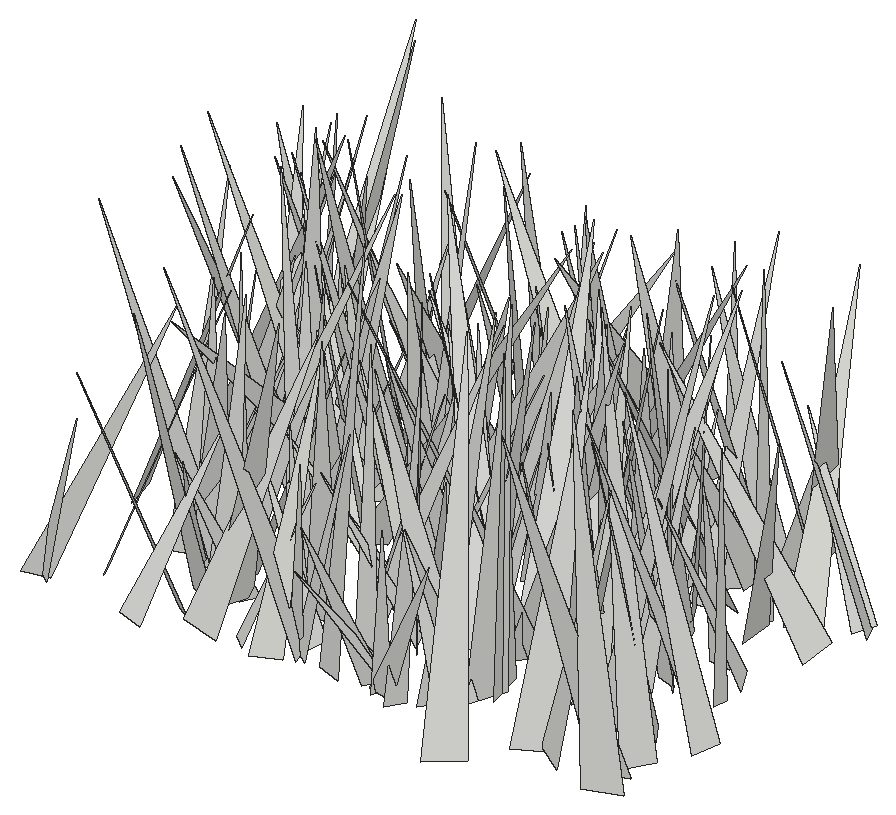
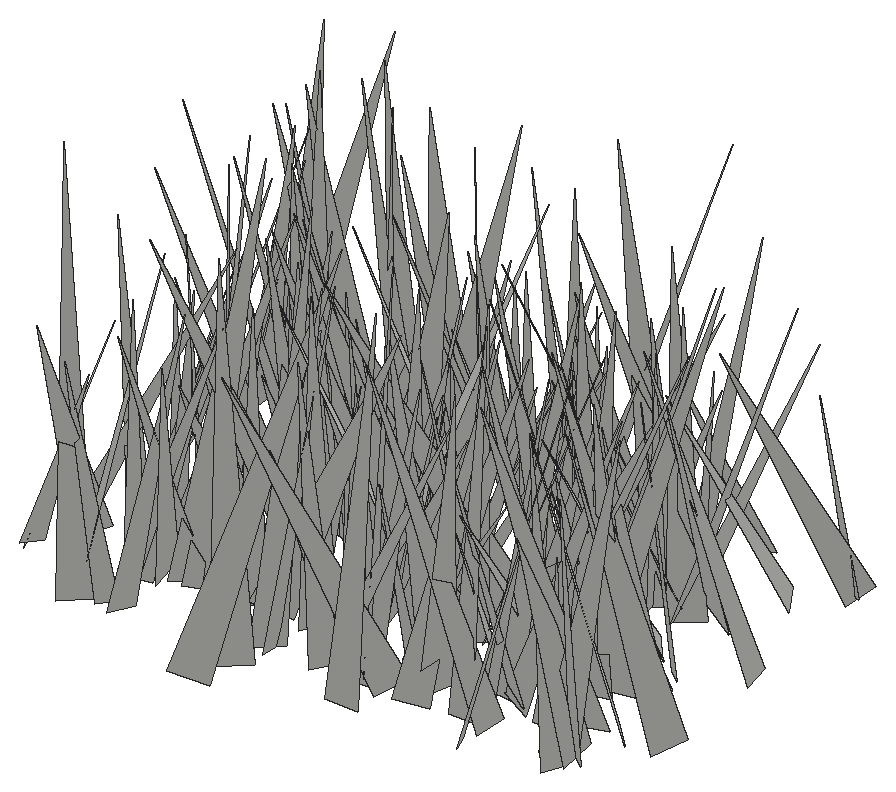
# SketchUp Ruby script. Lengths in inches.
U = 1.inch
M = Sketchup.active_model
def pt(a) = Geom::Point3d.new(a.map { |v| v * U })
def face(e, loops, mat)
  f = e.add_face(loops[0].map { |a| pt(a) })
  loops[1..].each { |l| e.add_face(l.map { |a| pt(a) }).erase! }
  f.material = f.back_material = mat if mat
  f
end
# faces: each face lists its corners as indices into pts; further lists are holes
def faces(e, pts, list, mat = nil) = list.each { |f| face(e, (f[0].is_a?(Array) ? f : [f]).map { |l| l.map { |i| pts[i] } }, mat) }
# xy, xz, yz: faces in a plane at the given z, y or x. An outline is a flat list of corners, or four numbers for a rectangle; further outlines are holes
def ring(l) = l.size == 4 ? [[l[0], l[1]], [l[2], l[1]], [l[2], l[3]], [l[0], l[3]]] : l.each_slice(2).to_a
def flat(e, list, mat, &to3) = list.each { |f| face(e, (f[0].is_a?(Array) ? f : [f]).map { |l| ring(l).map { |u, v| to3.(u, v) } }, mat) }
def xy(e, z, list, mat = nil) = flat(e, list, mat) { |x, y| [x, y, z] }
def xz(e, y, list, mat = nil) = flat(e, list, mat) { |x, z| [x, y, z] }
def yz(e, x, list, mat = nil) = flat(e, list, mat) { |y, z| [x, y, z] }
def lines(e, pts, list) = list.each { |a, b| e.add_line(pt(pts[a]), pt(pts[b])) }
# prism: a flat outline (further loops are holes) pulled along v
def prism(e, loops, v, mat = nil)
  f = face(e, loops, mat); d = Geom::Vector3d.new(v.map { |x| x * U })
  f.pushpull(f.normal.samedirection?(d) ? d.length : -d.length)
end
def box(e, o, s, mat = nil) = prism(e, [[o, [o[0] + s[0], o[1], o[2]], [o[0] + s[0], o[1] + s[1], o[2]], [o[0], o[1] + s[1], o[2]]]], [0, 0, s[2]], mat)
def at(x, y, z, deg = 0) = Geom::Transformation.translation(pt([x, y, z])) * Geom::Transformation.rotation(ORIGIN, Z_AXIS, deg.degrees)
def axes(o, x, y, z) = Geom::Transformation.new([*x, 0, *y, 0, *z, 0, *pt(o).to_a, 1])
def part(name) = M.definitions.add(name)
# library, detail: a bought-in or finely detailed component or shape, given as its bounding box
def library(name, o, s) = part(name).tap { |d| box(d.entities, o, s) }
def detail(e, o, s) = box(e.add_group.entities, o, s)
def put(e, d, t, mat = nil) = e.add_instance(d, t).tap { |i| i.material = mat if mat }
def group(e, t, mat = nil) = e.add_group.tap { |g| g.transformation = t; g.material = mat if mat }.entities
root = M.entities
c1 = part("fur_instance\#9")
p = [[0.8125,0,1.79],[0.67,-0.02,1.48],[0,-0.11,0],[0,0.11,0]]
faces(c1.entities,p,[[0,1,2,3]])
put(root,c1,axes([494.21,43.57,-21.86],[-3.24466,-1.65637,0.06319],[-1.44148,2.88818,1.68993],[0.81834,-1.47993,3.2273]))
put(root,c1,axes([493.82,43.125,-21.86],[1.92833,-3.54748,0.58332],[-3.33012,-2.01195,-1.22706],[-1.35468,-0.10385,3.84674]))
put(root,c1,axes([504.59,43.15,-21.86],[0.14854,-7.36709,1.66817],[-7.40985,-0.46607,-1.39849],[-1.46661,1.60862,7.23466]))
put(root,c1,axes([479.7,41.96,-21.86],[2.1321,2.91958,1.28602],[3.18698,-1.87905,-1.01782],[0.14466,-1.63367,3.46899]))
put(root,c1,axes([494.51,42.625,-21.86],[1.15805,-3.96128,0.43832],[-3.70743,-0.90324,1.63219],[1.46246,0.84697,3.79062]))
put(root,c1,axes([505.06,42.02,-21.86],[1.15068,-6.84996,3.27998],[-7.48842,-1.57649,-0.66528],[-1.26644,3.09791,6.914]))
put(root,c1,axes([490.3,43.63,-21.86],[-7.76303,-2.55675,1.09489],[-2.43873,7.81802,0.96517],[1.33728,-0.58482,8.11604]))
put(root,c1,axes([485.34,42.9,-21.86],[-3.10953,-4.00727,0.37973],[-3.98696,3.00024,-0.98706],[-0.55366,0.90108,4.97525]))
put(root,c1,axes([494.37,42.82,-21.86],[3.31226,-1.52366,0.97308],[-1.49474,-3.45052,-0.31491],[-1.01694,0.10903,3.63228]))
put(root,c1,axes([499.3,40.25,-21.86],[5.53383,-2.65462,5.00816],[-4.23304,-6.59023,1.18414],[-3.76962,3.5034,6.0223]))
put(root,c1,axes([484.17,41.32,-21.86],[0.26684,4.21608,0.5662],[4.07293,-0.08948,-1.25314],[1.22767,-0.6195,4.03438]))
put(root,c1,axes([497.21,43.58,-21.86],[4.68158,-4.31782,3.21331],[-4.18207,-5.59908,-1.43065],[-3.3881,0.94493,6.20597]))
put(root,c1,axes([496.99,44.51,-21.86],[4.08531,-1.79648,1.28746],[-1.24322,-4.1049,-1.78292],[-1.82737,-1.22355,4.09124]))
put(root,c1,axes([485.21,44.25,-21.86],[-2.27159,-6.08211,1.19958],[-6.16809,2.34544,0.21162],[0.62109,1.04786,6.48903]))
put(root,c1,axes([502.05,42.74,-21.86],[3.01267,4.99828,1.819],[5.31773,-2.78497,-1.15474],[0.11548,-2.15148,5.72063]))
put(root,c1,axes([486.27,44.47,-21.86],[7.12513,-3.29011,0.44393],[-3.26274,-7.13377,-0.50321],[-0.6135,-0.27186,7.83192]))
put(root,c1,axes([490.04,43.42,-21.86],[-1.12295,-3.74744,1.45837],[-3.89173,1.39395,0.58526],[1.01223,1.20198,3.86805]))
put(root,c1,axes([486.59,42.27,-21.86],[0.24671,6.36494,1.6516],[6.30189,0.24313,-1.87833],[1.87786,-1.65213,6.08648]))
put(root,c1,axes([488.23,42.47,-21.86],[2.19151,2.85606,0.09461],[2.85445,-2.18225,-0.24214],[0.13471,-0.22234,3.59182]))
put(root,c1,axes([490.47,43.09,-21.86],[2.5994,3.80823,1.24151],[3.99906,-2.55122,-0.54734],[-0.2268,-1.33772,4.57819]))
put(root,c1,axes([479.54,41.77,-21.86],[5.30796,-1.91017,1.71118],[-2.50762,-4.68997,2.54311],[-0.53734,3.01775,5.03546]))
put(root,c1,axes([483.86,45.68,-21.86],[4.12034,-0.14152,0.59374],[0.17297,-3.61498,-2.06197],[-0.58535,-2.06437,3.57009]))
put(root,c1,axes([486.6,45.11,-21.86],[1.61464,-3.26071,0.69447],[-2.99454,-1.75765,-1.29032],[-1.46534,-0.00102,3.40211]))
put(root,c1,axes([489.68,42.16,-21.86],[-4.32625,3.6169,1.13686],[3.35652,4.45591,-1.40339],[1.76301,0.39209,5.46158]))
put(root,c1,axes([490.55,44.03,-21.86],[-3.79909,0.62191,0.11225],[0.62576,3.79759,0.13861],[0.08831,-0.15497,3.84716]))
put(root,c1,axes([495.39,42.34,-21.86],[-6.05732,0.47074,1.68041],[-0.07648,5.99257,-1.95441],[1.74342,1.89841,5.75265]))
put(root,c1,axes([501.28,42.81,-21.86],[-4.71435,5.59524,2.23508],[5.56124,5.13291,-1.11952],[2.31839,-0.93486,7.23039]))
put(root,c1,axes([489.55,45.53,-21.86],[0.93072,-6.54849,1.55591],[-6.7031,-0.75944,0.81335],[0.60996,1.64631,6.5641]))
put(root,c1,axes([492.14,42.65,-21.86],[3.45024,7.01244,2.07893],[6.95776,-3.8555,1.45774],[-2.25516,-1.1667,7.67811]))
put(root,c1,axes([489.56,44.42,-21.86],[0.08392,3.77547,1.67654],[4.10941,-0.2474,0.35143],[-0.42151,-1.66031,3.76001]))
put(root,c1,axes([497.6,44.75,-21.86],[7.52534,-2.11015,2.94691],[-2.32099,-8.02168,0.183],[-2.78389,0.98374,7.81345]))
put(root,c1,axes([496.41,43.25,-21.86],[-6.74927,1.80081,2.69667],[1.18797,7.16726,-1.81295],[3.01723,1.2063,6.74602]))
put(root,c1,axes([497.76,45.6,-21.86],[-6.42267,-1.42598,3.31634],[-1.29179,7.22813,0.60623],[3.37087,0.05298,6.55107]))
put(root,c1,axes([483.23,47.04,-21.86],[3.73638,-5.69312,0.32255],[-5.69521,-3.70663,0.54933],[0.28337,0.57053,6.78752]))
put(root,c1,axes([493.14,46.59,-21.86],[-3.84083,-1.16764,0.10273],[-1.10793,3.73134,0.98769],[0.38264,-0.91633,3.89099]))
put(root,c1,axes([496.77,45.57,-21.86],[7.78387,0.2727,2.09642],[0.3333,-8.05673,-0.18953],[-2.08764,-0.26953,7.78634]))
put(root,c1,axes([492.2,44.7,-21.86],[1.00537,5.49165,1.69021],[5.63183,-1.28199,0.81538],[-1.13911,-1.49133,5.52306]))
put(root,c1,axes([493.0625,46.44,-21.86],[5.50119,4.10651,2.99111],[4.73487,-5.74232,-0.82461],[-1.84151,-2.49711,6.81516]))
put(root,c1,axes([481.34,43.51,-21.86],[4.7893,3.01055,0.30481],[2.77693,-4.59952,1.79634],[-1.20208,1.36921,5.36414]))
put(root,c1,axes([485.07,45.49,-21.86],[4.88657,-1.90502,2.44295],[-2.30886,-5.28158,0.49977],[-2.06549,1.39696,5.22091]))
put(root,c1,axes([503.95,46.5,-21.86],[-4.7875,-3.33897,1.34753],[-3.4677,4.87923,-0.23006],[0.96934,0.96392,5.83232]))
put(root,c1,axes([483.83,46.17,-21.86],[0.33576,5.45677,2.6197],[6.05197,-0.25349,-0.24764],[0.11336,-2.62894,5.46148]))
put(root,c1,axes([483.78,46.71,-21.86],[-7.05109,-1.52018,0.70264],[-1.52291,7.08527,0.04653],[0.69669,0.10238,7.21295]))
put(root,c1,axes([491.65,47.875,-21.86],[-4.59032,-0.23962,0.17171],[-0.16134,4.28449,1.66587],[0.24672,-1.65642,4.28408]))
put(root,c1,axes([505.12,47.69,-21.86],[-6.09562,-2.74651,0.83103],[-2.67616,6.14538,0.68045],[1.03541,-0.28555,6.65108]))
put(root,c1,axes([504.86,44.28,-21.86],[-8.1921,1.36867,0.61461],[1.20152,8.02801,-1.8625],[0.89853,1.74336,8.09413]))
put(root,c1,axes([497.72,47.76,-21.86],[-0.21744,-4.53269,0.61909],[-4.46943,0.07824,-0.99696],[-0.9761,0.65149,4.42703]))
put(root,c1,axes([484.6875,46.88,-21.86],[0.05129,-4.93553,2.34933],[-4.99892,0.90807,2.01684],[2.21125,2.16734,4.50493]))
put(root,c1,axes([491.35,45.6875,-21.86],[3.76049,3.04894,0.61025],[2.98388,-3.80785,0.6375],[-0.87456,0.11813,4.79905]))
put(root,c1,axes([491.22,46.125,-21.86],[3.55811,5.92159,0.8478],[5.93377,-3.36884,-1.37307],[0.75783,-1.4247,6.77052]))
put(root,c1,axes([497.4,50.3,-21.86],[1.43301,-8.2393,0.15598],[-8.02359,-1.35888,1.93375],[1.87948,0.48092,8.13635]))
put(root,c1,axes([506.01,46.69,-21.86],[-6.67851,0.63047,0.27765],[0.60623,6.66388,-0.54986],[0.32721,0.52189,6.68563]))
put(root,c1,axes([485.01,46.55,-21.86],[-5.66532,-0.50223,1.85308],[-0.88322,5.80808,-1.12609],[1.70472,1.34012,5.57494]))
put(root,c1,axes([485.65,46.37,-21.86],[4.63443,1.21877,0.59299],[1.09033,-4.6073,0.94811],[-0.80513,0.77609,4.69728]))
put(root,c1,axes([496.93,47.83,-21.86],[7.07738,-3.29601,0.99897],[-3.4049,-7.03943,0.89669],[-0.51794,1.23844,7.75557]))
put(root,c1,axes([492.52,47.16,-21.86],[5.45999,3.37552,0.2587],[3.37248,-5.38033,-0.97518],[0.29572,-0.96459,6.34466]))
put(root,c1,axes([498.69,49.59,-21.86],[1.50872,-5.62418,0.24688],[-5.60162,-1.47433,0.64555],[0.56049,0.40439,5.78713]))
put(root,c1,axes([491.5,49.68,-21.86],[-0.15941,-4.26775,0.08772],[-3.87813,0.18147,1.78158],[1.78369,0.01316,3.88138]))
put(root,c1,axes([492.75,49.84,-21.86],[1.73584,-5.70606,0.92261],[-5.63591,-1.88469,-1.0526],[-1.28332,0.55882,5.87063]))
put(root,c1,axes([502.09,45.85,-21.86],[3.85814,7.37241,1.12129],[7.37277,-3.96052,0.67189],[-1.11889,-0.67587,8.29374]))
put(root,c1,axes([493.59,51.07,-21.86],[-5.30348,-5.59312,0.1785],[-5.55783,5.29332,0.73008],[0.65218,-0.37354,7.67313]))
put(root,c1,axes([487.97,46.46,-21.86],[-7.72963,0.57294,0.92033],[0.30078,7.49944,-2.14251],[1.04153,2.08628,7.44883]))
put(root,c1,axes([491.89,48.14,-21.86],[-4.67921,0.76999,0.1435],[0.76372,4.67821,-0.1991],[0.17382,0.17327,4.73796]))
put(root,c1,axes([500.125,46.79,-21.86],[6.4621,3.38539,1.99868],[3.00841,-6.73382,1.67909],[-2.53082,0.63956,7.09931]))
put(root,c1,axes([484.01,46.44,-21.86],[4.66085,6.54813,0.11631],[6.5407,-4.64683,-0.4912],[0.3329,-0.37945,8.02249]))
put(root,c1,axes([485.61,53.69,-21.86],[5.32765,-5.22538,0.29084],[-4.03169,-4.36253,-4.52625],[-3.33686,-3.07194,5.93309]))
put(root,c1,axes([482.48,46.23,-21.86],[2.16067,6.65454,0.44246],[6.23565,-2.18071,2.34697],[-2.36543,0.32979,6.59114]))
put(root,c1,axes([495.39,47.69,-21.86],[-5.00695,6.61488,0.9269],[6.67749,4.92855,0.89773],[-0.16413,-1.27989,8.24744]))
put(root,c1,axes([478.77,48.67,-21.86],[6.39935,1.66924,0.57136],[1.67346,-6.42366,0.02366],[-0.55885,-0.12123,6.61343]))
put(root,c1,axes([486.08,50.76,-21.86],[1.95757,-4.55386,0.31612],[-4.56359,-1.94437,0.25034],[0.10577,0.38911,4.95045]))
put(root,c1,axes([494.55,48.66,-21.86],[-0.54447,5.56352,1.73211],[5.79599,0.33809,0.73596],[-0.59958,-1.78391,5.54144]))
put(root,c1,axes([501.86,49.64,-21.86],[-2.15143,-4.58063,1.63472],[-4.86135,2.07952,-0.57094],[0.14745,1.72526,5.02841]))
put(root,c1,axes([496.65,49.89,-21.86],[-1.9321,-3.03286,0.9193],[-3.13143,1.99261,-0.00754],[0.48737,0.77951,3.596]))
put(root,c1,axes([493.47,50.32,-21.86],[3.99613,2.0991,0.80323],[2.24013,-3.58697,-1.77087],[0.18236,-1.93595,4.15203]))
put(root,c1,axes([501.96,49.77,-21.86],[4.37424,4.04681,2.79179],[4.54542,-4.75288,-0.23239],[-1.87347,-2.08284,5.95454]))
put(root,c1,axes([484.71,50.74,-21.86],[-7.47727,-2.4998,1.10622],[-2.44373,7.5564,0.55783],[1.22512,-0.18436,7.86431]))
put(root,c1,axes([495.05,48.03,-21.86],[-1.19348,5.65379,0.3473],[5.3271,0.99964,2.033],[-1.92561,-0.73875,5.40894]))
put(root,c1,axes([503.95,51.41,-21.86],[-4.09527,-2.1175,0.66115],[-1.87882,4.04889,1.32991],[1.17939,-0.90267,4.41434]))
put(root,c1,axes([485.18,50.01,-21.86],[5.23095,-0.44242,1.6949],[-0.413,-5.49862,-0.16069],[-1.70231,-0.02548,5.24716]))
put(root,c1,axes([482.97,52.85,-21.86],[-1.44964,-7.72306,0.36058],[-7.72764,1.4358,-0.315],[-0.24346,0.41228,7.85162]))
put(root,c1,axes([481.11,50.42,-21.86],[3.62429,3.41254,1.71474],[3.78655,-3.51895,-1.00013],[-0.49783,-1.92166,4.87654]))
put(root,c1,axes([497.43,52.25,-21.86],[5.27759,-3.33069,0.22963],[-3.2336,-5.20637,-1.19863],[-0.83073,-0.89406,6.12452]))
put(root,c1,axes([488.09,50.05,-21.86],[-3.65286,-4.07637,1.60167],[-4.37583,3.48496,-1.11027],[0.18514,1.94004,5.3598]))
put(root,c1,axes([499.88,47.99,-21.86],[0.68594,6.83231,0.78357],[6.74689,-0.82108,1.2531],[-1.33188,-0.64057,6.75135]))
put(root,c1,axes([501.44,48.8,-21.86],[1.25627,4.75609,0.70963],[4.78282,-1.31187,0.32531],[-0.49861,-0.60066,4.90844]))
put(root,c1,axes([496.32,50.91,-21.86],[-2.25784,-3.06403,1.232],[-3.11024,2.47464,0.4545],[1.1102,0.70132,3.77883]))
put(root,c1,axes([492.93,51.22,-21.86],[3.77255,3.78798,3.73229],[4.48771,-4.72284,0.25719],[-2.85294,-2.4201,5.33992]))
put(root,c1,axes([497.06,48.28,-21.86],[-3.53884,7.24303,1.02774],[7.25201,3.62348,-0.56563],[0.96238,-0.67082,8.04145]))
put(root,c1,axes([489.66,50.85,-21.86],[2.40925,-3.29701,1.00546],[-3.44676,-2.29271,0.74099],[0.03277,1.24857,4.01568]))
put(root,c1,axes([504.34,49.6,-21.86],[-4.48133,-0.60292,1.35721],[-0.97091,4.45413,-1.22715],[1.12377,1.44397,4.35201]))
put(root,c1,axes([496.25,52.36,-21.86],[6.83248,-2.68093,1.04491],[-2.55055,-6.88917,-0.99801],[-1.33189,-0.56029,7.27146]))
put(root,c1,axes([492.59,50.99,-21.86],[-3.18222,-1.83698,0.96818],[-1.93012,3.2701,-0.13938],[0.76583,0.60852,3.67173]))
put(root,c1,axes([486.72,48.33,-21.86],[4.61652,6.22378,1.13894],[6.03614,-4.75491,1.51682],[-1.89675,0.0163,7.59914]))
put(root,c1,axes([500.76,52.23,-21.86],[-6.30807,-3.21691,2.7037],[-2.95993,6.86307,1.25992],[2.98285,0.00727,6.96799]))
put(root,c1,axes([493.87,52.3,-21.86],[2.32363,-4.81619,0.47979],[-4.81966,-2.25368,0.71896],[0.44354,0.74187,5.29887]))
put(root,c1,axes([482.82,49.01,-21.86],[3.00596,2.69315,0.13963],[2.45938,-2.82346,1.51258],[-1.10635,1.04086,3.74179]))
put(root,c1,axes([502.57,51.8,-21.86],[0.0054,-4.02258,1.09842],[-4.16704,0.03516,0.14925],[0.15324,1.09787,4.01982]))
put(root,c1,axes([495.42,50.81,-21.86],[3.80415,1.70942,1.42934],[1.7089,-4.05302,0.29902],[-1.42996,-0.29602,4.15984]))
put(root,c1,axes([498.64,49.8,-21.86],[-4.20959,5.12778,0.85898],[5.1677,4.24809,-0.03415],[0.57165,-0.64206,6.63427]))
put(root,c1,axes([497.76,52.06,-21.86],[0.0044,-6.27087,2.13822],[-6.5778,-0.25997,-0.7489],[-0.79272,2.12236,6.226]))
put(root,c1,axes([491.73,52.17,-21.86],[2.95462,-6.48005,1.02046],[-5.97059,-2.19282,3.36242],[2.71745,2.2277,6.27814]))
put(root,c1,axes([493.55,50.37,-21.86],[2.79902,6.82497,1.56007],[7.00009,-2.70115,-0.74237],[0.11309,-1.72399,7.33919]))
put(root,c1,axes([498.92,49.92,-21.86],[1.72672,7.47142,1.23195],[7.48463,-1.49226,-1.44043],[1.14896,-1.50745,7.53186]))
put(root,c1,axes([488.33,52.99,-21.86],[4.8862,-3.80667,1.31151],[-3.74132,-5.05482,-0.73291],[-1.48774,0.20937,6.1505]))
put(root,c1,axes([497.57,50.16,-21.86],[-3.3116,2.69695,0.72945],[2.42136,3.33487,-1.33716],[1.39378,0.61437,4.05614]))
put(root,c1,axes([483.55,51.9375,-21.86],[2.46407,-3.91283,1.91735],[-4.25122,-2.64198,0.07181],[-0.95581,1.66367,4.6235]))
put(root,c1,axes([485.42,52.12,-21.86],[-7.85705,-0.88135,0.16267],[-0.88597,7.85465,-0.23661],[0.1352,0.25331,7.90278]))
put(root,c1,axes([480.39,51.51,-21.86],[3.49532,2.40186,0.16337],[2.40303,-3.46356,-0.49202],[0.14512,-0.49771,4.21237]))
put(root,c1,axes([484.21,52.49,-21.86],[1.0853,-7.02468,2.48253],[-7.23303,-0.3918,2.05344],[1.78669,2.68091,6.80495]))
put(root,c1,axes([488.28,51.87,-21.86],[-6.99068,-2.50094,0.47101],[-2.54423,6.83653,-1.46112],[-0.05835,1.53405,7.27938]))
put(root,c1,axes([479.74,52.96,-21.86],[1.22983,-5.08709,1.30795],[-5.046,-0.77126,1.74491],[1.45845,1.62123,4.93419]))
put(root,c1,axes([487.375,50.91,-21.86],[7.21653,-2.33327,0.39687],[-2.31249,-6.67999,2.77668],[0.50399,2.75925,7.05779]))
put(root,c1,axes([482.56,53.32,-21.86],[1.05516,-7.50337,2.43147],[-7.87164,-0.84629,0.8044],[0.49989,2.51181,7.53438]))
put(root,c1,axes([482.93,49.03,-21.86],[4.07419,5.57288,0.07978],[5.18286,-3.82462,2.48447],[-2.04971,1.40628,6.44076]))
put(root,c1,axes([486.57,51.16,-21.86],[-3.04335,5.85133,0.32291],[5.70958,2.87864,1.64877],[-1.32023,-1.03909,6.38604]))
put(root,c1,axes([502.17,54.33,-21.86],[5.73315,-1.08828,0.33068],[-0.98004,-5.58896,-1.40205],[-0.57725,-1.3198,5.66459]))
put(root,c1,axes([499.96,55.35,-21.86],[-1.99035,-6.59495,0.1128],[-6.59501,1.99173,0.07994],[0.10913,0.08488,6.88828]))
put(root,c1,axes([489.75,53,-21.86],[4.40599,-6.63506,1.39046],[-6.52465,-3.70025,3.01783],[1.84021,2.76664,7.37085]))
put(root,c1,axes([484.27,51.2,-21.86],[-0.89857,4.82904,0.37817],[4.8418,0.88433,0.21213],[-0.14006,-0.41036,4.90735]))
put(root,c1,axes([485.59,53.36,-21.86],[3.00214,-3.52749,1.91618],[-3.65397,-3.39209,-0.51969],[-1.66236,1.08552,4.60282]))
put(root,c1,axes([498.93,51.75,-21.86],[2.68485,5.08236,0.90598],[5.15716,-2.6868,-0.21076],[-0.23424,-0.9002,5.74408]))
put(root,c1,axes([479.61,52.88,-21.86],[5.01329,4.55618,1.17415],[4.70331,-4.80639,-1.43108],[0.12753,-1.84671,6.62147]))
put(root,c1,axes([492.79,50.52,-21.86],[4.99959,5.18328,0.38062],[5.01525,-4.9501,1.53324],[-1.36326,0.79826,7.03643]))
put(root,c1,axes([500.43,51.18,-21.86],[-3.90191,2.21296,0.38649],[1.88444,3.64598,-1.85127],[1.22289,1.44261,4.08594]))
put(root,c1,axes([492.07,53.85,-21.86],[-1.04898,-5.12431,2.12616],[-5.35306,1.50327,0.98203],[1.45734,1.83333,5.13756]))
put(root,c1,axes([504.74,54.59,-21.86],[-6.59727,0.97904,0.29915],[1.02311,6.37288,1.70633],[0.03533,-1.73199,6.44755]))
put(root,c1,axes([495.3,53.72,-21.86],[2.23095,-4.80055,1.901],[-5.14348,-2.24733,0.36107],[-0.45138,1.8816,5.28129]))
put(root,c1,axes([485.1,55.33,-21.86],[-0.40917,-7.70862,1.45343],[-7.84037,0.35495,-0.32469],[-0.25296,1.46762,7.71264]))
put(root,c1,axes([499.71,53.85,-21.86],[5.0794,2.90769,2.21904],[3.29641,-5.28463,-0.62087],[-1.58507,-1.67247,5.81975]))
put(root,c1,axes([495.57,52.09,-21.86],[-5.59441,-0.96055,0.72122],[-1.15543,5.24244,-1.98041],[0.32833,2.08191,5.31959]))
put(root,c1,axes([488.38,55.67,-21.66],[2.87814,-5.28951,1.31735],[-4.95416,-3.15966,-1.86304],[-2.27391,0.18887,5.72641]))
put(root,c1,axes([492.08,53.55,-21.86],[-3.98181,3.20015,0.16473],[3.12043,3.81261,1.36007],[-0.7287,-1.16015,4.92402]))
put(root,c1,axes([491.6,53.1875,-21.86],[-5.02924,-0.94611,0.83871],[-1.10156,4.96734,-1.00192],[0.62059,1.14984,5.01842]))
put(root,c1,axes([481.87,52.59,-21.86],[-1.61925,6.67608,1.38838],[6.8184,1.60284,0.24489],[0.08425,-1.4073,6.86528]))
put(root,c1,axes([498.55,56,-21.66],[6.46231,-4.31648,2.52967],[-3.92803,-6.93665,-1.8017],[-3.09867,-0.20881,7.55958]))
put(root,c1,axes([481.68,51.73,-21.86],[2.76869,6.15296,0.77217],[6.00563,-2.8712,1.34513],[-1.54517,-0.13446,6.61174]))
put(root,c1,axes([487.64,55.63,-21.66],[2.89446,-5.47209,0.08006],[-5.31049,-2.7865,1.53693],[1.32243,0.78724,5.99662]))
put(root,c1,axes([498.28,56.3,-21.66],[4.1039,-1.37964,0.4984],[-1.03776,-3.77714,-1.91052],[-1.03675,-1.68037,3.88527]))
put(root,c1,axes([496.34,53.69,-21.86],[1.80379,6.11401,2.80003],[6.29213,-2.55743,1.53087],[-2.37284,-2.13386,6.18799]))
put(root,c1,axes([489.17,51.55,-21.86],[3.53249,6.50702,1.2231],[6.07163,-3.73652,2.34297],[-2.64057,0.11331,7.02355]))
put(root,c1,axes([478.01,54.55,-21.86],[7.43524,-1.67911,0.29476],[-1.69435,-7.42416,0.44731],[-0.18841,0.50147,7.60934]))
put(root,c1,axes([482.43,56.11,-21.86],[-0.97227,-5.54065,0.71566],[-5.53732,1.05209,0.62249],[0.741,0.5921,5.59077]))
put(root,c1,axes([491.96,54.96,-21.86],[4.11916,-1.93041,1.42636],[-1.9279,-4.34864,-0.31782],[-1.42975,0.30221,4.53795]))
put(root,c1,axes([488.25,54.96,-21.86],[1.60844,-3.68609,1.55705],[-3.78668,-1.94455,-0.69177],[-1.29334,1.10916,3.96179]))
put(root,c1,axes([489.57,54.84,-21.86],[-2.45268,-3.25533,0.28731],[-3.08329,2.18606,-1.55237],[-1.08306,1.14864,3.76868]))
put(root,c1,axes([495.99,55.71,-21.86],[4.8037,-2.51399,0.9877],[-2.43404,-4.90267,-0.64073],[-1.17095,-0.12226,5.38379]))
put(root,c1,axes([486.94,58.05,-21.66],[5.11337,-4.37567,0.02712],[-4.08728,-4.79107,-2.37351],[-1.56248,-1.78687,6.29758]))
put(root,c1,axes([484.35,52.77,-21.86],[3.84867,2.11329,0.22175],[1.92609,-3.66331,1.48248],[-0.8974,1.20066,4.13285]))
put(root,c1,axes([484.24,55.51,-21.86],[-2.37076,-5.83706,1.32394],[-5.9146,2.06646,-1.48049],[-0.91737,1.76156,6.12372]))
put(root,c1,axes([500.02,57.01,-21.66],[4.14247,-2.36814,0.94959],[-1.79033,-3.98803,-2.13546],[-1.81783,-1.46881,4.26707]))
put(root,c1,axes([493.75,54.17,-21.86],[7.5928,-1.32868,0.07278],[-1.31152,-7.40102,1.71058],[0.22497,1.69728,7.51598]))
put(root,c1,axes([485.1,55.9,-21.86],[-4.49464,-4.79472,1.8462],[-5.03521,4.59856,-0.3156],[1.02201,1.56958,6.56442]))
put(root,c1,axes([497.26,55.14,-21.86],[4.42317,-1.03576,2.17466],[-1.28949,-4.85884,0.30856],[-2.03449,0.82776,4.53233]))
put(root,c1,axes([489.51,57.22,-21.66],[6.5233,2.37968,3.04495],[3.30026,-6.53866,-1.96019],[-2.01069,-3.01183,6.66138]))
put(root,c1,axes([493.49,57.97,-21.66],[7.48346,-2.4752,1.75576],[-1.96533,-7.51292,-2.21472],[-2.31232,-1.62508,7.56464]))
put(root,c1,axes([485.14,57.46,-21.86],[-1.97553,-6.78705,1.45707],[-6.65434,2.28292,1.61176],[1.97656,0.90224,6.88251]))
put(root,c1,axes([493.21,55.42,-21.86],[-5.47966,3.19166,2.7493],[3.39794,6.01513,-0.2105],[2.48986,-1.18473,6.33791]))
put(root,c1,axes([486.51,53.62,-21.86],[2.91558,3.30379,0.88214],[2.68077,-2.92801,2.10571],[-2.12289,0.83996,3.8706]))
put(root,c1,axes([489.24,57.75,-21.86],[-0.08674,-5.50292,0.32115],[-5.49794,0.10952,0.39174],[0.3974,0.31411,5.48965]))
put(root,c1,axes([494.87,56.9,-21.86],[-1.51621,-3.26203,0.55212],[-3.23761,1.58793,0.49084],[0.68086,0.28668,3.56354]))
put(root,c1,axes([488.54,55.85,-21.86],[3.55375,0.65284,0.74182],[0.70307,-3.6162,-0.18565],[-0.69441,-0.32026,3.60844]))
put(root,c1,axes([484.22,55.41,-21.86],[2.56604,4.25646,1.10853],[4.39439,-2.42581,-0.85772],[0.18887,-1.38883,4.89555]))
put(root,c1,axes([495.21,55.61,-21.86],[-4.31341,6.46311,1.11663],[6.32564,3.74609,2.75266],[-1.73345,-2.41229,7.26637]))
put(root,c1,axes([482.03,56.04,-21.86],[-3.27969,0.65416,1.38528],[0.68941,3.5533,-0.04576],[1.36808,-0.22237,3.34398]))
put(root,c1,axes([493.08,54.73,-21.86],[4.03542,0.28371,1.50858],[-0.2798,-4.0361,1.5075],[-1.50932,1.50677,3.754]))
put(root,c1,axes([479.85,54.94,-21.86],[4.5925,4.65986,1.11021],[4.70947,-4.6734,0.13435],[-0.87619,-0.69491,6.5412]))
put(root,c1,axes([493.24,58.14,-21.66],[-5.97447,-2.65496,2.2585],[-2.10106,6.3191,1.8704],[2.78122,-0.92951,6.26456]))
put(root,c1,axes([480.8,57.375,-21.86],[3.4747,-4.84053,2.29693],[-4.84614,-4.00697,-1.11322],[-2.28507,1.13736,5.85363]))
put(root,c1,axes([501.93,55.02,-21.86],[-6.28866,-0.36775,1.68536],[-0.82762,6.23312,-1.72806],[1.51351,1.8804,6.05775]))
put(root,c1,axes([483.79,59.2,-21.66],[-5.87667,-3.9224,1.1719],[-3.54254,5.90008,1.98324],[2.05159,-1.04767,6.78139]))
put(root,c1,axes([505.3,56.89,-21.86],[-4.74174,-2.50609,0.51828],[-2.55748,4.67952,-0.77105],[0.09149,0.92453,5.30754]))
put(root,c1,axes([491.22,57.61,-21.86],[4.9839,-2.53795,0.76874],[-2.53211,-5.04073,-0.2255],[-0.78777,0.14572,5.58834]))
put(root,c1,axes([500.93,59.6,-21.66],[8.00988,-2.00577,0.3429],[-1.833,-7.71682,-2.32157],[-0.88363,-2.17404,7.92412]))
put(root,c1,axes([494.23,61.54,-21.66],[6.48177,-5.01878,0.45242],[-4.24735,-5.8379,-3.90962],[-2.71162,-2.85253,7.2053]))
put(root,c1,axes([480.27,58.29,-21.86],[6.05752,-0.57817,0.88939],[-0.39,-6.0087,-1.2499],[-0.9865,-1.17476,5.9553]))
put(root,c1,axes([501.74,58.51,-21.86],[-4.76298,-4.61729,1.21885],[-4.61962,4.89113,0.47635],[1.20999,0.49843,6.61653]))
put(root,c1,axes([491.01,57.41,-21.66],[-4.07281,-4.5818,0.7427],[-4.55178,3.7491,-1.83244],[-0.90871,1.75604,5.85003]))
put(root,c1,axes([500.3,57.5,-21.66],[-2.82559,-5.19892,1.36333],[-5.31081,2.46391,-1.61114],[-0.82624,1.9421,5.69358]))
put(root,c1,axes([504.97,56.97,-21.86],[-3.82314,1.91513,0.41484],[1.95484,3.79049,0.51675],[0.13566,-0.64863,4.24466]))
put(root,c1,axes([483.89,57.35,-21.86],[7.09843,0.26187,0.16049],[0.26265,-7.10014,-0.03187],[-0.15921,-0.03777,7.10319]))
put(root,c1,axes([487.03,56.46,-21.86],[-6.58758,2.43197,1.48528],[2.355,6.75255,-0.6115],[1.60454,0.07391,6.99549]))
put(root,c1,axes([499.44,54.72,-21.86],[1.20703,6.81999,0.05967],[6.70849,-1.19813,1.23829],[-1.22962,0.158,6.81439]))
put(root,c1,axes([481.2,55.2,-21.86],[-1.14842,8.02715,0.79991],[8.02073,1.22255,-0.75306],[0.86188,-0.68125,8.07384]))
put(root,c1,axes([493.86,59.56,-21.86],[5.04429,-5.44094,0.7168],[-5.46997,-5.06343,0.05905],[-0.44381,0.56596,7.41924]))
put(root,c1,axes([480.2,57.04,-21.86],[7.83085,1.1219,1.78667],[1.00117,-8.02181,0.64907],[-1.85702,0.40616,7.88414]))
put(root,c1,axes([480.24,57.12,-21.86],[2.88835,4.68484,1.93004],[4.79823,-3.24275,0.69058],[-1.62782,-1.24585,5.46016]))
put(root,c1,axes([500.14,58.77,-21.86],[1.41621,-4.16021,0.5332],[-4.01988,-1.18575,1.42542],[1.19673,0.94019,4.15706]))
put(root,c1,axes([489.01,59.39,-21.86],[-0.69172,-7.26259,1.83893],[-7.46362,0.82804,0.46276],[0.64909,1.78171,7.28077]))
put(root,c1,axes([499.59,56.04,-21.66],[-6.16922,0.32467,1.04524],[-0.06119,5.87189,-2.18505],[1.09279,2.16166,5.77844]))
put(root,c1,axes([499.45,58.82,-21.86],[-5.83631,0.9789,1.84731],[1.28037,6.00401,0.86359],[1.65271,-1.19453,5.85448]))
put(root,c1,axes([488.17,57.58,-21.66],[4.70359,-4.43483,0.77561],[-4.1988,-3.91632,3.07011],[1.62462,2.71804,5.6891]))
put(root,c1,axes([503.48,55.375,-21.66],[-5.02723,4.35262,0.08247],[4.19421,4.87628,-1.68986],[1.1665,1.22544,6.43138]))
